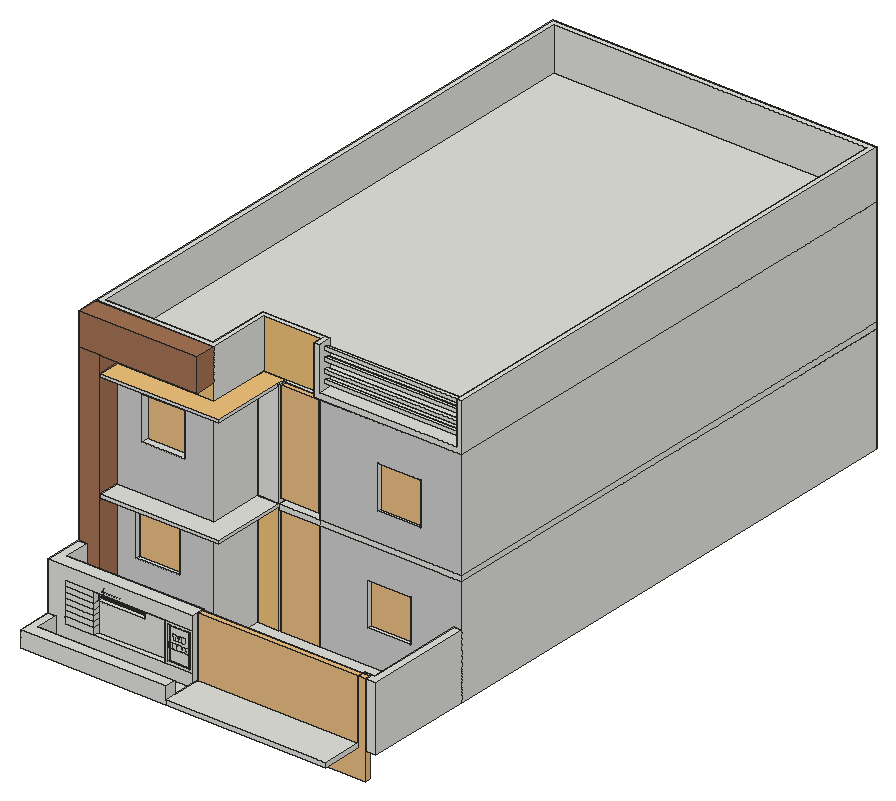
# SketchUp Ruby script. Lengths in inches.
U = 1.inch
M = Sketchup.active_model
def pt(a) = Geom::Point3d.new(a.map { |v| v * U })
def face(e, loops, mat)
  f = e.add_face(loops[0].map { |a| pt(a) })
  loops[1..].each { |l| e.add_face(l.map { |a| pt(a) }).erase! }
  f.material = f.back_material = mat if mat
  f
end
# faces: each face lists its corners as indices into pts; further lists are holes
def faces(e, pts, list, mat = nil) = list.each { |f| face(e, (f[0].is_a?(Array) ? f : [f]).map { |l| l.map { |i| pts[i] } }, mat) }
# xy, xz, yz: faces in a plane at the given z, y or x. An outline is a flat list of corners, or four numbers for a rectangle; further outlines are holes
def ring(l) = l.size == 4 ? [[l[0], l[1]], [l[2], l[1]], [l[2], l[3]], [l[0], l[3]]] : l.each_slice(2).to_a
def flat(e, list, mat, &to3) = list.each { |f| face(e, (f[0].is_a?(Array) ? f : [f]).map { |l| ring(l).map { |u, v| to3.(u, v) } }, mat) }
def xy(e, z, list, mat = nil) = flat(e, list, mat) { |x, y| [x, y, z] }
def xz(e, y, list, mat = nil) = flat(e, list, mat) { |x, z| [x, y, z] }
def yz(e, x, list, mat = nil) = flat(e, list, mat) { |y, z| [x, y, z] }
def lines(e, pts, list) = list.each { |a, b| e.add_line(pt(pts[a]), pt(pts[b])) }
# prism: a flat outline (further loops are holes) pulled along v
def prism(e, loops, v, mat = nil)
  f = face(e, loops, mat); d = Geom::Vector3d.new(v.map { |x| x * U })
  f.pushpull(f.normal.samedirection?(d) ? d.length : -d.length)
end
def box(e, o, s, mat = nil) = prism(e, [[o, [o[0] + s[0], o[1], o[2]], [o[0] + s[0], o[1] + s[1], o[2]], [o[0], o[1] + s[1], o[2]]]], [0, 0, s[2]], mat)
def at(x, y, z, deg = 0) = Geom::Transformation.translation(pt([x, y, z])) * Geom::Transformation.rotation(ORIGIN, Z_AXIS, deg.degrees)
def axes(o, x, y, z) = Geom::Transformation.new([*x, 0, *y, 0, *z, 0, *pt(o).to_a, 1])
def part(name) = M.definitions.add(name)
# library, detail: a bought-in or finely detailed component or shape, given as its bounding box
def library(name, o, s) = part(name).tap { |d| box(d.entities, o, s) }
def detail(e, o, s) = box(e.add_group.entities, o, s)
def put(e, d, t, mat = nil) = e.add_instance(d, t).tap { |i| i.material = mat if mat }
def group(e, t, mat = nil) = e.add_group.tap { |g| g.transformation = t; g.material = mat if mat }.entities
root = M.entities
M.materials.add("[Carrera Marble]").color = [207, 207, 207]
M.materials.add("[Tile Ceramic Multi]").color = [165, 115, 84]
M.materials.add("[Wood OSB]").color = [240, 195, 122]
c1 = library("Untitled",[72.44,-487.65,0],[104,4,82])
c2 = part("TEJU KUMAR")
xy(c2.entities,0.03,[[7.1875,0,6.71,0.03,6.31,0.13,5.98,0.3,5.74,0.53,5.55,0.84,5.42,1.24,5.34,1.73,5.3125,2.3125,5.3125,5.84,6.64,5.84,6.64,1.84,6.68,1.59,6.79,1.39,6.96,1.27,7.1875,1.23,7.42,1.27,7.6,1.41,7.71,1.61,7.75,1.89,7.75,5.84,9.07,5.84,9.07,2.11,9.02,1.43,8.87,0.89,8.62,0.49,8.28,0.22,7.81,0.05],[0.82,0.16,0.82,5.84,2.11,5.84,2.11,3.17,2.13,3.17,3.35,5.84,4.71,5.84,3.39,2.9375,4.65,0.16,3.23,0.16,2.13,2.52,2.11,2.52,2.11,0.16],[10.03,0.16,10.65,5.84,12.28,5.84,12.83,2.68,12.97,3.56,13.15,4.56,13.4,5.84,15.07,5.84,15.71,0.16,14.4375,0.16,14.09,4.07,13.29,0.16,12.42,0.16,11.59,4.08,11.25,0.16],[[16.25,0.16,17.75,5.84,19.2,5.84,20.71,0.16,19.37,0.16,19.15,1.11,17.79,1.11,17.5625,0.16],[18.02,2.13,18.9,2.13,18.65,3.37,18.47,4.54,18.45,4.54,18.27,3.35]],[[21.36,0.16,21.36,5.84,22.86,5.84,23.29,5.8125,23.68,5.73,24.01,5.58,24.3,5.375,24.53,5.12,24.7,4.82,24.8,4.48,24.83,4.1,24.78,3.69,24.63,3.3,24.38,2.96,24.05,2.72,25.08,0.16,23.71,0.16,22.67,2.75,22.65,2.75,22.65,0.16],[22.65,3.39,23.02,3.4375,23.29,3.55,23.45,3.74,23.51,3.99,23.46,4.33,23.31,4.5625,23.04,4.69,22.65,4.74]],
  [13.28,10.05,12.86,10.11,12.44,10.29,12.44,11.58,12.78,11.39,13,11.33,13.22,11.37,13.37,11.48,13.46,11.68,13.49,11.95,13.49,15.9,14.78,15.9,14.78,11.81,14.76,11.43,14.68,11.1,14.55,10.8,14.37,10.54,14.15,10.33,13.89,10.17,13.61,10.08],[17.81,10.05,17.33,10.09,16.93,10.1875,16.6,10.35,16.35,10.58,16.17,10.89,16.04,11.29,15.96,11.78,15.93,12.37,15.93,15.9,17.26,15.9,17.26,11.89,17.29,11.64,17.41,11.45,17.58,11.33,17.81,11.28,18.04,11.33,18.22,11.46,18.33,11.67,18.37,11.94,18.37,15.9,19.68,15.9,19.68,12.17,19.63,11.48,19.48,10.94,19.24,10.55,18.89,10.27,18.43,10.11],[6.24,10.21,6.24,14.6,5.36,14.6,5.36,15.9,8.44,15.9,8.44,14.6,7.55,14.6,7.55,10.21],[9.24,10.21,9.24,15.9,11.85,15.9,11.85,14.6875,10.53,14.6875,10.53,13.64,11.68,13.64,11.68,12.46,10.53,12.46,10.53,11.43,11.86,11.43,11.86,10.21]])
c3 = library("cancello1",[20.57,-4.21,-37.54],[271.95,5,121.42])
c4 = library("porta 4",[0.2,-5.42,1.33],[46.55,4.72,83.21])
xy(root,0,[[9,13.49,161.375,38.1875],[0,38.1875,9,80.75],[9,38.1875,9,53.26,155.57,53.26,155.57,44.75,161.375,44.75,161.375,38.1875],[161.62,44.75,161.375,53.26,9,53.26,9,80.75,0,80.75,0,104.75,132,104.75,132,164.75,156,164.75,156,173.75,123,173.75,123,113.75,9,113.75,9,104.75,0,104.75,0,740.75,360,740.75,360,164.75,351,164.75,351,53.97,339.875,53.97,339.875,44.75],[155.57,44.75,155.57,53.26,161.22,53.26,161.375,50.02,161.375,44.75],
  [161.375,44.75,161.375,50.02,161.62,44.75],[161.62,44.75,161.375,50.02,161.375,53.26],[339.875,44.75,339.875,53.97,351,53.97,351,164.75,360,164.75,360,44.75],[161.375,50.02,161.22,53.26,161.375,53.26],[9,104.75,9,113.75,123,113.75,123,173.75,132,173.75,132,104.75],
  [132,164.75,156,173.75]])
xy(root,5.1875,[[161.375,0,340.25,44.75]])
xy(root,13.96,[[51.11,38.1875,130.31,44.75]])
xy(root,17.04,[[133.38,38.1875,158.3,48.625]])
xy(root,18.5625,[[0,0,161.375,0,161.375,13.49,9,13.49,9,38.1875,0,38.1875]])
xy(root,18.65,[[134.99,38.6875,156.69,48.625]])
xy(root,37.02,[[254.74,164.75,302.74,173.75]])
xy(root,45.53,[[51,38.1875,51.11,44.75],[51,44.75,102.37,53.26]])
xy(root,52.91,[[134.99,38.6875,156.69,48.625]])
xy(root,54.52,[[133.38,38.1875,158.3,48.625]])
xy(root,57.59,[[51,38.1875,51,53.26,102.37,53.26,102.37,44.75,130.31,44.75,130.31,38.1875]])
xy(root,60.2,[[45.29,104.75,93.29,113.75]])
xy(root,72,[[0,38.1875,161.375,38.1875,161.375,53.26,9,53.26,9,80.75,0,80.75],[339.875,44.75,360,44.75,360,164.75,351,164.75,351,53.97,339.875,53.97]])
xy(root,85.02,[[254.74,164.75,302.74,173.75]])
xy(root,108.2,[[45.29,104.75,93.29,113.75]])
xy(root,120,[[0,113.75,9,740.75],[156,164.75,202,173.75],[202,164.75,351,173.75],[351,164.75,360,740.75],[9,731.75,351,740.75]])
xy(root,123,[[24,80.75,24,104.75,132,104.75,132,164.75,156.25,164.75,156.25,80.75]])
xy(root,126.4375,[[24,80.75,156.25,80.75,156.25,164.75,132,164.75,132,104.75,24,104.75],[9,113.75,123,113.75,123,173.75,156,173.75,156,164.75,202,164.75,202,173.75,351,173.75,351,731.75,9,731.75]])
xy(root,157.84,[[266.38,164.75,314.38,173.75]])
xy(root,178.1,[[51.71,104.75,99.71,113.75]])
xy(root,205.84,[[266.38,164.75,314.38,173.75]])
xy(root,226.1,[[51.71,104.75,99.71,113.75]])
xy(root,243.62,[[24,80.75,24,104.75,132,104.75,132,164.75,156,164.75,156,80.75]])
xy(root,246.4375,[[123,104.75,132,173.75],[0,113.75,9,740.75],[195,164.75,202,173.75],[202,164.75,351,173.75],[351,164.75,360,740.75],
  [9,731.75,351,740.75]])
xy(root,252.875,[[6,110.75,126,110.75,126,179.75,201,179.75,201,164.75,354,164.75,354,734.75,6,734.75]])
xy(root,259.47,[[201,171.21,353.75,175.27]])
xy(root,263.53,[[201,171.21,353.75,175.27]])
xy(root,270.16,[[201,171.21,354,175.27]])
xy(root,274.22,[[201,171.21,354,175.27]])
xy(root,281.53,[[201,171.21,354,175.27]])
xy(root,285.59,[[201,171.21,354,175.27]])
xy(root,292.28,[[201,171.21,357.5,175.27]])
xy(root,296.34,[[201,171.21,357.5,175.27]])
xy(root,300.875,[[0,104.75,132,104.75,132,173.75,195,173.75,195,179.75,126,179.75,126,110.75,6,110.75,6,734.75,354,734.75,354,164.75,360,164.75,360,740.75,0,740.75],[195,164.75,201,179.75]])
xz(root,0,[[0,0,161.375,18.5625],[161.375,0,340.25,5.1875]])
xz(root,13.49,[[9,0,161.375,18.5625]])
xz(root,38.1875,[[0,0,6,18.5625],[9,0,161.375,0,161.375,13.96,18.74,13.96,18.74,57.59,161.375,57.59,161.375,72,0,72,0,18.5625,9,18.5625],[6,0,9,18.5625],[18.74,13.96,51.11,21.48],[[130.31,13.96,161.375,57.59],[133.38,17.04,158.3,54.52]],
  [18.74,21.48,51.11,27.48],[18.74,27.48,51.11,33.48],[18.74,33.48,51.11,39.48],[18.74,39.48,51.11,39.48,51.11,45.53,51,45.53,51,45.7,18.74,45.7],[18.74,45.7,51,51.65],
  [18.74,51.65,51,57.59]])
xz(root,38.6875,[[134.99,18.65,156.69,52.91]])
xz(root,44.75,[[161.375,0,161.62,5.1875],[161.62,0,339.875,5.1875],[339.875,0,340.25,5.1875],[340.25,0,360,0,360,72,339.875,72,339.875,5.1875,340.25,5.1875],[51.11,13.96,130.31,13.96,130.31,57.59,102.37,57.59,102.37,45.53,51.11,45.53],
  [51,45.53,51.11,57.59]])
xz(root,48.625,[[[133.38,17.04,158.3,54.52],[134.99,18.65,156.69,52.91]]])
xz(root,53.26,[[[9,0,161.375,72],[51,45.53,102.37,57.59]]])
xz(root,53.97,[[339.875,0,351,72]])
xz(root,80.75,[[0,0,9,72],[24,123,156.25,126.4375]])
xz(root,104.75,[[[24,0,132,123],[45.29,60.2,93.29,108.2]],[[24,126.4375,132,243.62],[51.71,178.1,99.71,226.1]]],"[Carrera Marble]")
xz(root,104.75,[[24,246.4375,132,264.875]],"[Wood OSB]")
xz(root,110.75,[[6,252.875,126,300.875]])
xz(root,113.75,[[[9,0,123,120],[45.29,60.2,93.29,108.2]],[[9,126.4375,123,246.4375],[51.71,178.1,99.71,226.1]]])
xz(root,164.75,[[351,0,360,72],[156,120,156.25,123],[156.25,120,202,126.4375],[202,120,360,126.4375],[132,123,156,126.4375],
  [156,123,156.25,126.4375],[132,126.4375,156,243.62],[195,246.4375,360,246.4375,360,300.875,354,300.875,354,252.875,201,252.875,201,300.875,195,300.875]])
xz(root,164.75,[[[202,0,351,0,351,72,360,72,360,120,202,120],[254.74,37.02,302.74,85.02]],[[202,126.4375,360,246.4375],[266.38,157.84,314.38,205.84]]],"[Carrera Marble]")
xz(root,164.75,[[132,0,156,123]],"[Wood OSB]")
xz(root,171.21,[[201,259.47,353.75,263.53],[201,270.16,354,274.22],[201,281.53,354,285.59],[201,292.28,357.5,296.34]])
xz(root,173.75,[[123,0,132,120],[132,0,156,120],[132,120,156,126.4375],[123,126.4375,132,246.4375],[132,126.4375,156,246.4375],
  [[202,126.4375,351,246.4375],[266.38,157.84,314.38,205.84]]])
xz(root,173.75,[[132,246.4375,195,300.875]],"[Wood OSB]")
xz(root,175.27,[[201,259.47,353.75,263.53],[201,270.16,354,274.22],[201,281.53,354,285.59],[201,292.28,357.5,296.34]])
xz(root,179.75,[[126,252.875,195,300.875],[195,252.875,201,300.875]])
xz(root,731.75,[[9,0,351,120],[9,126.4375,351,246.4375]])
xz(root,734.75,[[6,252.875,354,300.875]])
xz(root,740.75,[[0,0,360,120],[0,120,360,126.4375],[0,126.4375,360,246.4375],[0,246.4375,360,300.875]])
yz(root,0,[[0,0,38.1875,18.5625],[38.1875,0,80.75,72],[104.75,0,740.75,120],[104.75,120,740.75,126.4375],[104.75,126.4375,740.75,246.4375],
  [104.75,246.4375,740.75,300.875]])
yz(root,6,[[110.75,252.875,734.75,300.875]])
yz(root,9,[[13.49,0,38.1875,18.5625],[53.26,0,80.75,72],[113.75,0,731.75,120],[113.75,126.4375,731.75,246.4375]])
yz(root,24,[[80.75,123,104.75,126.4375],[80.75,243.62,104.75,246.4375]])
yz(root,45.29,[[104.75,60.2,113.75,108.2]])
yz(root,51,[[38.1875,45.53,44.75,45.7],[[44.75,45.53,53.26,57.59],[48.88,53.81,48.625,53.84,48.38,53.94,48.18,54.1,48.02,54.31,47.92,54.55,47.88,54.81,47.92,55.07,48.02,55.31,48.18,55.51,48.38,55.67,48.625,55.77,48.88,55.81,49.14,55.77,49.38,55.67,49.59,55.51,49.75,55.31,49.85,55.07,49.88,54.81,49.85,54.55,49.75,54.31,49.59,54.1,49.38,53.94,49.14,53.84],[48.88,50.06,48.625,50.09,48.38,50.19,48.18,50.35,48.02,50.56,47.92,50.8,47.88,51.06,47.92,51.32,48.02,51.56,48.18,51.76,48.38,51.92,48.625,52.02,48.88,52.06,49.14,52.02,49.38,51.92,49.59,51.76,49.75,51.56,49.85,51.32,49.88,51.06,49.85,50.8,49.75,50.56,49.59,50.35,49.38,50.19,49.14,50.09],[48.88,47.06,48.625,47.09,48.38,47.19,48.18,47.35,48.02,47.56,47.92,47.8,47.88,48.06,47.92,48.32,48.02,48.56,48.18,48.76,48.38,48.92,48.625,49.02,48.88,49.06,49.14,49.02,49.38,48.92,49.59,48.76,49.75,48.56,49.85,48.32,49.88,48.06,49.85,47.8,49.75,47.56,49.59,47.35,49.38,47.19,49.14,47.09]],[38.1875,45.7,44.75,57.59]])
yz(root,51.11,[[38.1875,13.96,44.75,21.48],[38.1875,21.48,44.75,27.48],[38.1875,27.48,44.75,33.48],[38.1875,33.48,44.75,39.48],[38.1875,39.48,44.75,45.53]])
yz(root,51.71,[[104.75,178.1,113.75,226.1]])
yz(root,93.29,[[104.75,60.2,113.75,108.2]])
yz(root,99.71,[[104.75,178.1,113.75,226.1]])
yz(root,102.37,[[[44.75,45.53,53.26,57.59],[48.88,47.06,49.14,47.09,49.38,47.19,49.59,47.35,49.75,47.56,49.85,47.8,49.88,48.06,49.85,48.32,49.75,48.56,49.59,48.76,49.38,48.92,49.14,49.02,48.88,49.06,48.625,49.02,48.38,48.92,48.18,48.76,48.02,48.56,47.92,48.32,47.88,48.06,47.92,47.8,48.02,47.56,48.18,47.35,48.38,47.19,48.625,47.09],[48.88,50.06,49.14,50.09,49.38,50.19,49.59,50.35,49.75,50.56,49.85,50.8,49.88,51.06,49.85,51.32,49.75,51.56,49.59,51.76,49.38,51.92,49.14,52.02,48.88,52.06,48.625,52.02,48.38,51.92,48.18,51.76,48.02,51.56,47.92,51.32,47.88,51.06,47.92,50.8,48.02,50.56,48.18,50.35,48.38,50.19,48.625,50.09]]])
yz(root,104.25,[[48.88,53.81,49.14,53.84,49.38,53.94,49.59,54.1,49.75,54.31,49.85,54.55,49.88,54.81,49.85,55.07,49.75,55.31,49.59,55.51,49.38,55.67,49.14,55.77,48.88,55.81,48.625,55.77,48.38,55.67,48.18,55.51,48.02,55.31,47.92,55.07,47.88,54.81,47.92,54.55,48.02,54.31,48.18,54.1,48.38,53.94,48.625,53.84]])
yz(root,123,[[113.75,0,173.75,120],[113.75,126.4375,173.75,246.4375]])
yz(root,126,[[110.75,252.875,179.75,300.875]])
yz(root,130.31,[[38.1875,13.96,44.75,57.59]])
yz(root,132,[[104.75,0,164.75,123],[164.75,0,173.75,120],[164.75,120,173.75,126.4375],[104.75,126.4375,164.75,243.62],[164.75,126.4375,173.75,246.4375],
  [104.75,246.4375,173.75,300.875]])
yz(root,133.38,[[38.1875,17.04,48.625,54.52]])
yz(root,134.99,[[38.6875,18.65,48.625,52.91]])
yz(root,156,[[164.75,0,173.75,120],[164.75,120,173.75,126.4375],[164.75,126.4375,173.75,246.4375]])
yz(root,156.25,[[80.75,123,164.75,126.4375]])
yz(root,156.69,[[38.6875,18.65,48.625,52.91]])
yz(root,158.3,[[38.1875,17.04,48.625,54.52]])
yz(root,161.375,[[13.49,0,38.1875,5.1875],[38.1875,0,44.75,5.1875],[44.75,0,53.26,0,53.26,72,38.1875,72,38.1875,5.1875,44.75,5.1875],[0,5.1875,13.49,18.5625]])
yz(root,195,[[164.75,246.4375,173.75,300.875]])
yz(root,201,[[[164.75,252.875,179.75,300.875],[171.21,292.28,175.27,296.34],[171.21,281.53,175.27,285.59],[171.21,270.16,175.27,274.22],[171.21,259.47,175.27,263.53]]])
yz(root,202,[[164.75,0,173.75,120],[164.75,126.4375,173.75,246.4375]])
yz(root,254.74,[[164.75,37.02,173.75,85.02]])
yz(root,266.38,[[164.75,157.84,173.75,205.84]])
yz(root,302.74,[[164.75,37.02,173.75,85.02]])
yz(root,314.38,[[164.75,157.84,173.75,205.84]])
yz(root,339.875,[[44.75,0,53.97,72]])
yz(root,340.25,[[0,0,44.75,5.1875]])
yz(root,351,[[53.97,0,164.75,72],[173.75,0,731.75,120],[173.75,126.4375,731.75,246.4375]])
yz(root,353.75,[[171.21,259.47,175.27,263.53]])
yz(root,354,[[[164.75,252.875,734.75,300.875],[171.21,281.53,175.27,285.59],[171.21,270.16,175.27,274.22]]])
yz(root,357.5,[[171.21,292.28,175.27,296.34]])
yz(root,360,[[44.75,0,164.75,72],[164.75,0,740.75,120],[164.75,120,740.75,126.4375],[164.75,126.4375,740.75,246.4375],[164.75,246.4375,740.75,300.875]])
p = [[161.62,44.75,0],[161.375,53.26,0],[161.375,53.26,72],[161.62,44.75,72],[161.62,44.75,5.1875],[51,48.38,47.19],
  [51,48.625,47.09],[102.37,48.625,47.09],[102.37,48.38,47.19],[51,48.88,47.06],[102.37,48.88,47.06],[51,49.14,47.09],
  [102.37,49.14,47.09],[51,49.38,47.19],[102.37,49.38,47.19],[51,48.18,47.35],[102.37,48.18,47.35],[51,49.59,47.35],
  [102.37,49.59,47.35],[51,48.02,47.56],[102.37,48.02,47.56],[51,49.75,47.56],[102.37,49.75,47.56],[51,47.92,47.8],
  [102.37,47.92,47.8],[51,49.85,47.8],[102.37,49.85,47.8],[51,47.88,48.06],[102.37,47.88,48.06],[51,49.88,48.06],
  [102.37,49.88,48.06],[51,47.92,48.32],[102.37,47.92,48.32],[51,49.85,48.32],[102.37,49.85,48.32],[51,48.02,48.56],
  [102.37,48.02,48.56],[51,49.75,48.56],[102.37,49.75,48.56],[51,48.18,48.76],[102.37,48.18,48.76],[51,49.59,48.76],
  [102.37,49.59,48.76],[51,48.38,48.92],[102.37,48.38,48.92],[51,49.38,48.92],[102.37,49.38,48.92],[51,48.625,49.02],
  [102.37,48.625,49.02],[51,49.14,49.02],[102.37,49.14,49.02],[51,48.88,49.06],[102.37,48.88,49.06],[51,48.38,50.19],
  [51,48.625,50.09],[102.37,48.625,50.09],[102.37,48.38,50.19],[51,48.88,50.06],[102.37,48.88,50.06],[51,49.14,50.09],
  [102.37,49.14,50.09],[51,49.38,50.19],[102.37,49.38,50.19],[51,48.18,50.35],[102.37,48.18,50.35],[51,49.59,50.35],
  [102.37,49.59,50.35],[51,48.02,50.56],[102.37,48.02,50.56],[51,49.75,50.56],[102.37,49.75,50.56],[51,47.92,50.8],
  [102.37,47.92,50.8],[51,49.85,50.8],[102.37,49.85,50.8],[51,47.88,51.06],[102.37,47.88,51.06],[51,49.88,51.06],
  [102.37,49.88,51.06],[51,47.92,51.32],[102.37,47.92,51.32],[51,49.85,51.32],[102.37,49.85,51.32],[51,48.02,51.56],
  [102.37,48.02,51.56],[51,49.75,51.56],[102.37,49.75,51.56],[51,48.18,51.76],[102.37,48.18,51.76],[51,49.59,51.76],
  [102.37,49.59,51.76],[51,48.38,51.92],[102.37,48.38,51.92],[51,49.38,51.92],[102.37,49.38,51.92],[51,48.625,52.02],
  [102.37,48.625,52.02],[51,49.14,52.02],[102.37,49.14,52.02],[51,48.88,52.06],[102.37,48.88,52.06],[51,48.38,53.94],
  [51,48.625,53.84],[104.25,48.625,53.84],[104.25,48.38,53.94],[51,48.88,53.81],[104.25,48.88,53.81],[51,49.14,53.84],
  [104.25,49.14,53.84],[51,49.38,53.94],[104.25,49.38,53.94],[51,48.18,54.1],[104.25,48.18,54.1],[51,49.59,54.1],
  [104.25,49.59,54.1],[51,48.02,54.31],[104.25,48.02,54.31],[51,49.75,54.31],[104.25,49.75,54.31],[51,47.92,54.55],
  [104.25,47.92,54.55],[51,49.85,54.55],[104.25,49.85,54.55],[51,47.88,54.81],[104.25,47.88,54.81],[51,49.88,54.81],
  [104.25,49.88,54.81],[51,47.92,55.07],[104.25,47.92,55.07],[51,49.85,55.07],[104.25,49.85,55.07],[51,48.02,55.31],
  [104.25,48.02,55.31],[51,49.75,55.31],[104.25,49.75,55.31],[51,48.18,55.51],[104.25,48.18,55.51],[51,49.59,55.51],
  [104.25,49.59,55.51],[51,48.38,55.67],[104.25,48.38,55.67],[51,49.38,55.67],[104.25,49.38,55.67],[51,48.625,55.77],
  [104.25,48.625,55.77],[51,49.14,55.77],[104.25,49.14,55.77],[51,48.88,55.81],[104.25,48.88,55.81],[132,173.75,252.875],
  [132,179.75,252.875],[9,113.75,120],[9,104.75,120],[123,113.75,120],[123,104.75,120],[9,113.75,246.4375],
  [9,104.75,246.4375],[17.6,44.75,45.7],[18.74,44.75,45.7],[17.6,44.75,39.48],[18.74,44.75,39.48],[17.6,44.75,33.48],
  [18.74,44.75,33.48],[17.6,44.75,27.48],[18.74,44.75,27.48],[17.6,44.75,21.48],[18.74,44.75,21.48],[0,-34.9375,0],
  [9,-34.9375,0]]
faces(root,p,[[0,1,2,3,4],[5,6,7,8],[6,9,10,7],[9,11,12,10],[11,13,14,12],[15,5,8,16],[13,17,18,14],[19,15,16,20],
  [17,21,22,18],[23,19,20,24],[21,25,26,22],[27,23,24,28],[25,29,30,26],[31,27,28,32],[29,33,34,30],[35,31,32,36],
  [33,37,38,34],[39,35,36,40],[37,41,42,38],[43,39,40,44],[41,45,46,42],[47,43,44,48],[45,49,50,46],[51,47,48,52],
  [49,51,52,50],[53,54,55,56],[54,57,58,55],[57,59,60,58],[59,61,62,60],[63,53,56,64],[61,65,66,62],[67,63,64,68],
  [65,69,70,66],[71,67,68,72],[69,73,74,70],[75,71,72,76],[73,77,78,74],[79,75,76,80],[77,81,82,78],[83,79,80,84],
  [81,85,86,82],[87,83,84,88],[85,89,90,86],[91,87,88,92],[89,93,94,90],[95,91,92,96],[93,97,98,94],[99,95,96,100],
  [97,99,100,98],[101,102,103,104],[102,105,106,103],[105,107,108,106],[107,109,110,108],[111,101,104,112],[109,113,114,110],[115,111,112,116],
  [113,117,118,114],[119,115,116,120],[117,121,122,118],[123,119,120,124],[121,125,126,122],[127,123,124,128],[125,129,130,126],[131,127,128,132],
  [129,133,134,130],[135,131,132,136],[133,137,138,134],[139,135,136,140],[137,141,142,138],[143,139,140,144],[141,145,146,142],[147,143,144,148],
  [145,147,148,146]])
lines(root,p,[[149,150],[151,152],[153,154],[155,156],[157,158],[159,160],[161,162],[163,164],[165,166],[167,168]])
put(root,c1,axes([203.79,-1827.75,37.63],[0.6,0,0],[0,-4.128,0],[0,0,0.852]))
put(root,c1,axes([219.4375,-1828.06,157.68],[0.6,0,0],[0,-4.128,0],[0,0,0.852]))
put(root,c1,axes([7.04,-1883.78,177.89],[0.6,0,0],[0,-4.128,0],[0,0,0.852]))
put(root,c1,axes([2.55,-1887.5,43.07],[0.6,0,0],[0,-4.128,0],[0,0,0.852]))
put(root,c2,axes([134.11,38.6875,31.1],[0.912,0,0],[0,0,0.912],[0,-0.912,0]))
put(root,c3,axes([147.36,50.45,1.22],[0.6864,0,0],[0,1.35401,0],[0,0,0.84393]))
g1 = group(root,at(0,104.75,264.875),"[Tile Ceramic Multi]")
box(g1,[0,-24,0],[132,24,36])
g2 = group(root,at(18.74,44.75,13.96))
xz(g2,0,[[0,0,32.37,0,32.37,31.57,32.26,31.57,32.26,43.63,0,43.63]])
g3 = group(root,at(24,80.75,246.4375),"[Wood OSB]")
xy(g3,0,[[0,0,132,0,132,93,108,93,108,24,0,24]])
g4 = group(root,at(24,80.75,243.62))
xz(g4,0,[[0,0,132,2.82]])
g5 = group(root,at(156,80.75,243.62))
yz(g5,0,[[0,0,84,2.82]])
g6 = group(root,at(0,104.75,0),"[Tile Ceramic Multi]")
prism(g6,[[[24,-24,0],[24,-24,120],[24,-24,126.4375],[24,-24,246.4375],[24,-24,264.875],[0,-24,264.875],[0,-24,246.4375],[0,-24,126.4375],[0,-24,120],[0,-24,0],[9,-24,0]]],[0,24,0])
put(g6,c4,axes([158.37,58.42,131.67],[0.92,0,0],[0,-1.2604,0],[0,0,1.3524]))
put(g6,c4,axes([157.51,59.22,-4.21],[0.9384,0,0],[0,-1.11244,0],[0,0,1.46934]))
